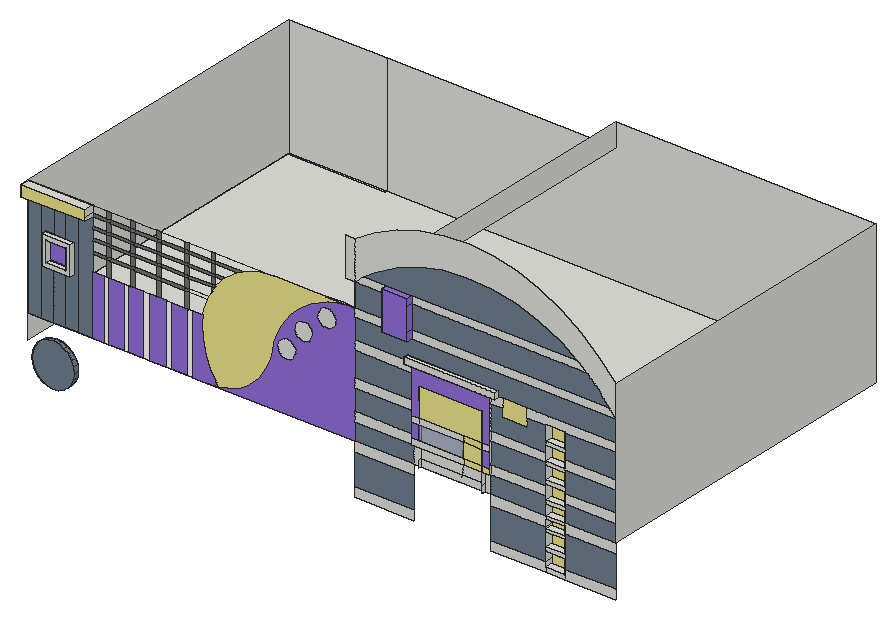
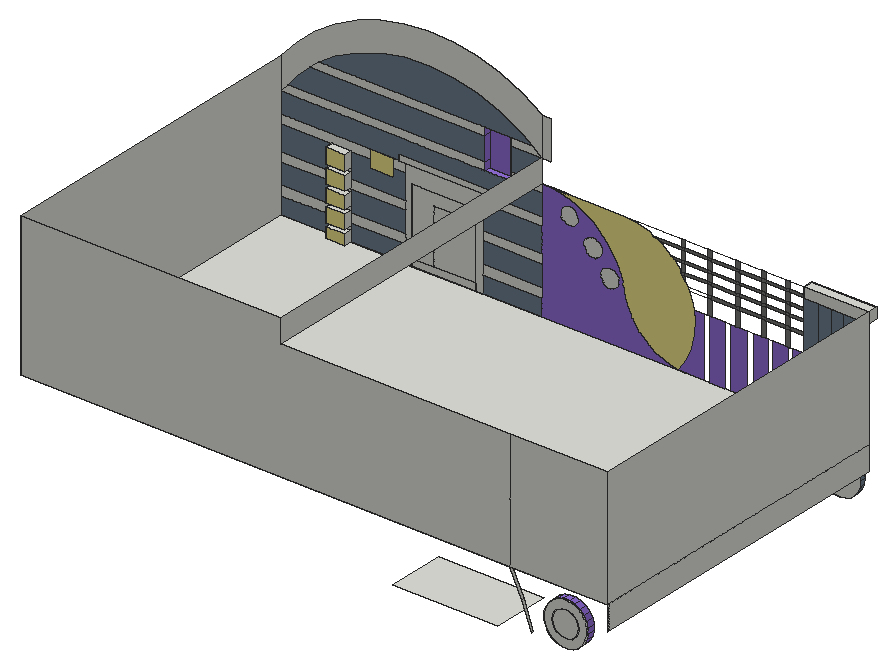
# SketchUp Ruby script. Lengths in inches.
U = 1.inch
M = Sketchup.active_model
def pt(a) = Geom::Point3d.new(a.map { |v| v * U })
def face(e, loops, mat)
  f = e.add_face(loops[0].map { |a| pt(a) })
  loops[1..].each { |l| e.add_face(l.map { |a| pt(a) }).erase! }
  f.material = f.back_material = mat if mat
  f
end
# faces: each face lists its corners as indices into pts; further lists are holes
def faces(e, pts, list, mat = nil) = list.each { |f| face(e, (f[0].is_a?(Array) ? f : [f]).map { |l| l.map { |i| pts[i] } }, mat) }
# xy, xz, yz: faces in a plane at the given z, y or x. An outline is a flat list of corners, or four numbers for a rectangle; further outlines are holes
def ring(l) = l.size == 4 ? [[l[0], l[1]], [l[2], l[1]], [l[2], l[3]], [l[0], l[3]]] : l.each_slice(2).to_a
def flat(e, list, mat, &to3) = list.each { |f| face(e, (f[0].is_a?(Array) ? f : [f]).map { |l| ring(l).map { |u, v| to3.(u, v) } }, mat) }
def xy(e, z, list, mat = nil) = flat(e, list, mat) { |x, y| [x, y, z] }
def xz(e, y, list, mat = nil) = flat(e, list, mat) { |x, z| [x, y, z] }
def yz(e, x, list, mat = nil) = flat(e, list, mat) { |y, z| [x, y, z] }
def lines(e, pts, list) = list.each { |a, b| e.add_line(pt(pts[a]), pt(pts[b])) }
# prism: a flat outline (further loops are holes) pulled along v
def prism(e, loops, v, mat = nil)
  f = face(e, loops, mat); d = Geom::Vector3d.new(v.map { |x| x * U })
  f.pushpull(f.normal.samedirection?(d) ? d.length : -d.length)
end
def box(e, o, s, mat = nil) = prism(e, [[o, [o[0] + s[0], o[1], o[2]], [o[0] + s[0], o[1] + s[1], o[2]], [o[0], o[1] + s[1], o[2]]]], [0, 0, s[2]], mat)
def at(x, y, z, deg = 0) = Geom::Transformation.translation(pt([x, y, z])) * Geom::Transformation.rotation(ORIGIN, Z_AXIS, deg.degrees)
def axes(o, x, y, z) = Geom::Transformation.new([*x, 0, *y, 0, *z, 0, *pt(o).to_a, 1])
def part(name) = M.definitions.add(name)
# library, detail: a bought-in or finely detailed component or shape, given as its bounding box
def library(name, o, s) = part(name).tap { |d| box(d.entities, o, s) }
def detail(e, o, s) = box(e.add_group.entities, o, s)
def put(e, d, t, mat = nil) = e.add_instance(d, t).tap { |i| i.material = mat if mat }
def group(e, t, mat = nil) = e.add_group.tap { |g| g.transformation = t; g.material = mat if mat }.entities
root = M.entities
M.materials.add("[0047_Khaki]").color = [240, 230, 140]
M.materials.add("[0111_SlateGray]").color = [112, 128, 144]
M.materials.add("[0115_MediumPurple]").color = [147, 112, 219]
M.materials.add("[Metal Seamed]").color = [118, 119, 115]
M.materials.add("[Translucent Glass Sky Reflection]").color = [126, 138, 183]
M.materials["[Translucent Glass Sky Reflection]"].alpha = 0.52
xy(root,99,[[81.125,144.5625,119.5625,165.625]])
xy(root,101.3125,[[231.02,45.625,238.14,48.4375]])
xy(root,103.03,[[231.02,45.625,238.14,48.4375]])
xy(root,108.37,[[231.02,45.625,238.14,48.4375]])
xy(root,109.71,[[231.02,45.625,238.14,48.4375]])
xy(root,114.67,[[231.02,45.625,238.14,48.4375]])
xy(root,115.6875,[[231.02,45.625,238.14,48.4375]])
xy(root,118.98,[[231.02,45.625,238.14,48.4375]])
xy(root,120,[[208.5625,44.5625,208.57,44.5625,208.57,45.625],[40.75,45.625,40.75,164.9375,76.51,164.9375,76.51,165.625,256.75,165.625,256.75,45.625,238.14,45.625,238.14,48.4375,231.02,48.4375,231.02,45.625,211.0625,45.625,211.0625,45.9375,182.75,45.9375,182.75,45.625],[182.75,45.625,185.24,45.9375],[185.24,45.625,208.57,45.9375],[208.57,45.625,211.0625,45.9375],
  [231.02,45.625,238.14,48.4375],[40.75,164.9375,76.51,165.625]])
xy(root,123.89,[[231.02,45.625,238.14,48.4375]])
xy(root,125.21,[[231.02,45.625,238.14,48.4375]])
xy(root,130.42,[[231.02,45.625,238.14,48.4375]])
xy(root,131.8125,[[231.02,45.625,238.14,48.4375]])
xy(root,136.6,[[231.02,45.625,238.14,48.4375]])
xy(root,137.97,[[231.02,45.625,238.14,48.4375]])
xy(root,138.5625,[[47.13,43.75,57.71,45.625]])
xy(root,140.1,[[48.67,43.75,56.17,45.625]])
xy(root,143.12,[[231.02,45.625,238.14,48.4375]])
xy(root,144.5,[[231.02,45.625,238.14,48.4375]])
xy(root,147.02,[[185.24,44.5625,186.69,45.625],[186.69,44.5625,208.57,45.625]])
xy(root,147.6,[[48.67,43.75,56.17,45.625]])
xy(root,149.13,[[47.13,43.75,57.71,45.625]])
xy(root,150.125,[[231.02,45.625,238.14,48.4375]])
xy(root,152.8125,[[180.25,44.125,182.75,45.625],[182.75,44.125,211.0625,44.5625],[211.0625,44.125,213.6875,45.625],[182.75,44.5625,211.0625,45.625]])
xy(root,155.0625,[[180.25,44.125,213.6875,45.625]])
xy(root,160.89,[[172.4,43.5,181.8125,45.625]],"[0115_MediumPurple]")
xy(root,163.75,[[40.75,42,64.49,45.625]])
xy(root,175.1,[[172.4,43.5,181.8125,45.625]],"[0115_MediumPurple]")
xz(root,42,[[40.75,159.875,64.49,160.08,64.49,163.75,40.75,163.75]],"[0047_Khaki]")
xz(root,43.5,[[172.4,160.89,181.8125,175.1]],"[0115_MediumPurple]")
xz(root,43.75,[[[47.13,138.5625,57.71,149.13],[48.67,140.1,56.17,147.6]]])
xz(root,44,[[51.27,99.26,53.3125,99.52,55.22,100.3,56.85,101.54,58.11,103.17,58.91,105.0625,59.18,107.1,58.92,109.14,58.14,111.04,56.9,112.68,55.28,113.9375,53.38,114.73,51.34,115.01,49.3,114.75,47.4,113.97,45.76,112.73,44.51,111.1,43.71,109.21,43.43,107.17,43.69,105.13,44.47,103.23,45.72,101.59,47.34,100.33,49.24,99.54]],"[0111_SlateGray]")
xz(root,44.125,[[180.25,152.8125,213.6875,155.0625]])
xz(root,44.5625,[[208.5625,120,208.57,120,208.57,122.49],[182.75,126.91,201.68,128.95],[182.75,134.36,185.24,136.41],[185.24,134.36,201.68,136.41],[208.57,134.36,211.0625,136.41]])
xz(root,44.5625,[[201.68,126.91,208.57,128.95],[208.57,126.91,211.0625,128.95],[201.68,128.95,208.57,134.36],[201.68,134.36,208.57,136.41],[185.24,136.41,208.57,147.02]],"[0047_Khaki]")
xz(root,44.5625,[[182.75,128.95,185.24,134.36],[208.57,128.95,211.0625,134.36],[182.75,136.41,185.24,136.41,185.24,147.02,208.57,147.02,208.57,136.41,211.0625,136.41,211.0625,152.8125,182.75,152.8125]],"[0115_MediumPurple]")
xz(root,44.5625,[[185.24,128.95,201.68,134.36]],"[Translucent Glass Sky Reflection]")
xz(root,45.625,[[51.27,99.26,49.24,99.54,47.34,100.33,45.72,101.59,44.47,103.23,43.69,105.13,43.43,107.17,43.71,109.21,44.51,111.1,45.76,112.73,47.4,113.97,49.3,114.75,51.34,115.01,53.38,114.73,55.28,113.9375,56.9,112.68,58.14,111.04,58.92,109.14,59.18,107.1,58.91,105.0625,58.11,103.17,56.85,101.54,55.22,100.3,53.3125,99.52],[160.75,101.3125,182.75,104.75],[211.0625,101.3125,231.02,104.75],[231.02,101.3125,238.14,103.03],[238.14,101.3125,256.75,104.75],
  [231.02,108.37,238.14,109.71],[231.02,114.67,238.14,115.6875],[160.75,116.3125,182.75,120],[211.0625,116.3125,231.02,120],[238.14,116.3125,256.75,120],
  [231.02,118.98,238.14,120],[182.75,120,182.75,152.8125,211.0625,152.8125,211.0625,120,208.57,120,208.57,147.02,185.24,147.02,185.24,120],[185.24,120,208.57,122.49],[185.24,122.49,200.8,142.51],[200.8,122.49,208.57,122.49,208.57,147.02,185.24,147.02,185.24,142.51,200.8,142.51],
  [231.02,123.89,238.14,125.21],[160.75,126.3125,182.75,129.75],[211.0625,126.3125,231.02,129.75],[238.14,126.3125,256.75,129.75],[231.02,130.42,238.14,131.8125],
  [231.02,136.6,238.14,137.97],[160.75,137.54,182.75,140.75],[211.0625,137.54,231.02,140.75],[238.14,137.54,256.75,140.75],[135.67,138.07,136.53,138.14,137.35,138.43,138.06,138.92,138.62,139.58,138.98,140.36,139.14,141.21,139.07,142.08,138.78,142.89,138.28,143.6,137.625,144.16,136.84,144.53,135.99,144.68,135.13,144.61,134.32,144.32,133.61,143.83,133.05,143.17,132.68,142.39,132.52,141.54,132.59,140.67,132.88,139.86,133.375,139.15,134.04,138.59,134.82,138.22],
  [[47.13,138.5625,57.71,149.13],[48.67,140.1,56.17,147.6]],[231.02,143.12,238.14,144.5],[141.94,146.02,142.8,146.09,143.62,146.38,144.33,146.87,144.89,147.53,145.26,148.3125,145.41,149.16,145.34,150.03,145.05,150.84,144.56,151.55,143.9,152.11,143.11,152.48,142.26,152.63,141.4,152.5625,140.59,152.27,139.875,151.78,139.32,151.12,138.95,150.34,138.79,149.49,138.86,148.625,139.16,147.81,139.65,147.1,140.31,146.54,141.09,146.17],[160.75,149.875,182.75,149.875,182.75,152.8125,180.25,152.8125,180.25,153.11,160.75,153.11],[211.0625,149.875,215.22,149.875,215.22,153.11,213.6875,153.11,213.6875,152.8125,211.0625,152.8125],
  [224.28,149.875,231.02,149.875,231.02,150.125,238.14,150.125,238.14,149.875,256.75,149.875,256.75,153.11,224.28,153.11],[180.25,152.8125,213.6875,155.0625],[150.53,153.47,151.39,153.54,152.21,153.83,152.92,154.33,153.48,154.99,153.85,155.77,154,156.62,153.93,157.48,153.64,158.29,153.15,159,152.49,159.5625,151.71,159.93,150.85,160.09,149.99,160.02,149.18,159.73,148.47,159.23,147.91,158.57,147.54,157.79,147.38,156.94,147.46,156.08,147.75,155.26,148.24,154.55,148.9,153.99,149.68,153.625],[40.75,159.875,40.75,163.75,64.49,163.75,64.49,160.08,50.125,159.96,45.3125,159.91],[160.75,160.89,172.4,163.75],
  [256.75,160.89,256.75,172.375,250.84,179.0625,244.13,184.94,236.72,189.93,228.74,193.93,220.32,196.88,211.59,198.74,202.7,199.48,193.78,199.08,184.99,197.55,176.46,194.92,168.34,191.22,160.75,186.53,160.75,172.375,164.37,175.1,167.99,177.82,175.92,182.21,184.38,185.46,193.21,187.51,202.24,188.32,211.29,187.87,220.19,186.17,228.77,183.26,236.87,179.18,242.78,175.1,244.32,174.03,246.12,172.375,250.99,167.89,254.4,163.75],[181.8125,160.89,256.75,160.89,254.4,163.75,181.8125,163.75],[150.22,163.75,160.75,163.75,156.39,164.07,152.03,163.97],[157.5625,172.375,160.75,186.53],[160.75,172.375,172.4,172.375,172.4,175.1,164.37,175.1],
  [181.8125,172.375,246.12,172.375,244.32,174.03,242.78,175.1,181.8125,175.1]])
xz(root,45.625,[[110.92,120.18,113.78,120.74,116.56,121.64,119.2,122.89,121.66,124.47,123.9,126.34,125.89,128.48,127.59,130.85,128.98,133.42,130.04,136.14,130.74,138.97,131.08,141.875,132.22,144.96,133.67,147.91,135.43,150.68,137.47,153.26,139.78,155.6,142.32,157.69,145.0625,159.5,147.98,161.01,151.05,162.2,154.22,163.06,157.47,163.58,160.75,163.75,131.08,163.75,126.1,163.28,121.29,161.87,119.97,161.19,117.79,160.08,116.84,159.59,113.35,156.86,112.89,156.5,112.43,155.98,109.94,153.12,109.6,152.73,109.23,152.11,108.25,150.41,107.08,148.41,106.78,147.58,105.41,143.6875,105.14,141.875,104.67,138.74,104.87,133.74,106.01,128.86,108.05,124.29],[215.22,146.8,224.28,153.11]],"[0047_Khaki]")
xz(root,45.625,[[160.75,104.75,182.75,116.3125],[211.0625,104.75,231.02,116.3125],[238.14,104.75,256.75,116.3125],[40.75,120,45.3125,120,45.3125,159.91,40.75,159.875],[45.3125,120,50.125,120,50.125,138.5625,47.13,138.5625,47.13,149.13,50.125,149.13,50.125,159.96,45.3125,159.91],
  [50.125,120,54.25,138.5625],[54.25,120,64.49,120,64.49,160.08,50.125,159.96,50.125,149.13,57.71,149.13,57.71,138.5625,54.25,138.5625],[160.75,120,182.75,126.3125],[211.0625,120,231.02,126.3125],[238.14,120,256.75,126.3125],
  [160.75,129.75,182.75,137.54],[211.0625,129.75,231.02,137.54],[238.14,129.75,256.75,137.54],[160.75,140.75,182.75,149.875],[211.0625,140.75,231.02,140.75,231.02,149.875,224.28,149.875,224.28,146.8,215.22,146.8,215.22,149.875,211.0625,149.875],
  [238.14,140.75,256.75,149.875],[160.75,153.11,180.25,153.11,180.25,155.0625,213.6875,155.0625,213.6875,153.11,256.75,153.11,256.75,160.89,160.75,160.89],[160.75,163.75,172.4,172.375],[181.8125,163.75,254.4,163.75,250.99,167.89,246.12,172.375,181.8125,172.375],[164.37,175.1,242.78,175.1,236.87,179.18,228.77,183.26,220.19,186.17,211.29,187.87,202.24,188.32,193.21,187.51,184.38,185.46,175.92,182.21,167.99,177.82]],"[0111_SlateGray]")
xz(root,45.625,[[64.49,120,68.69,141.875],[70.54,120,75.76,141.875],[77.65,120,82.98,141.875],[85.49,120,91.4,141.875],[93.75,120,99.21,141.875],
  [101.45,120,108,120,110.92,120.18,108.05,124.29,106.01,128.86,104.87,133.74,104.67,138.74,105.14,141.875,101.45,141.875],[[108,120,160.75,120,160.75,163.75,157.47,163.58,154.22,163.06,151.05,162.2,147.98,161.01,145.0625,159.5,142.32,157.69,139.78,155.6,137.47,153.26,135.43,150.68,133.67,147.91,132.22,144.96,131.08,141.875,130.74,138.97,130.04,136.14,128.98,133.42,127.59,130.85,125.89,128.48,123.9,126.34,121.66,124.47,119.2,122.89,116.56,121.64,113.78,120.74,110.92,120.18],[150.53,153.47,149.68,153.625,148.9,153.99,148.24,154.55,147.75,155.26,147.46,156.08,147.38,156.94,147.54,157.79,147.91,158.57,148.47,159.23,149.18,159.73,149.99,160.02,150.85,160.09,151.71,159.93,152.49,159.5625,153.15,159,153.64,158.29,153.93,157.48,154,156.62,153.85,155.77,153.48,154.99,152.92,154.33,152.21,153.83,151.39,153.54],[135.67,138.07,134.82,138.22,134.04,138.59,133.375,139.15,132.88,139.86,132.59,140.67,132.52,141.54,132.68,142.39,133.05,143.17,133.61,143.83,134.32,144.32,135.13,144.61,135.99,144.68,136.84,144.53,137.625,144.16,138.28,143.6,138.78,142.89,139.07,142.08,139.14,141.21,138.98,140.36,138.62,139.58,138.06,138.92,137.35,138.43,136.53,138.14],[141.94,146.02,141.09,146.17,140.31,146.54,139.65,147.1,139.16,147.81,138.86,148.625,138.79,149.49,138.95,150.34,139.32,151.12,139.875,151.78,140.59,152.27,141.4,152.5625,142.26,152.63,143.11,152.48,143.9,152.11,144.56,151.55,145.05,150.84,145.34,150.03,145.41,149.16,145.26,148.3125,144.89,147.53,144.33,146.87,143.62,146.38,142.8,146.09]],[48.67,140.1,56.17,147.6]],"[0115_MediumPurple]")
xz(root,45.625,[[69.84,141.875,71.23,147.58],[78.54,141.875,80,147.58],[88,141.875,89.49,147.58],[98.4,141.875,100.02,147.58],[64.49,147.58,69.84,148.74],
  [69.84,147.58,71.23,148.74],[71.23,147.58,78.54,148.74],[78.54,147.58,80,148.74],[80,147.58,88,148.74],[88,147.58,89.49,148.74],
  [89.49,147.58,98.4,148.74],[98.4,147.58,100.02,148.74],[69.84,148.74,71.23,152.11],[78.54,148.74,80,152.11],[88,148.74,89.49,152.11],
  [98.4,148.74,100.02,152.11],[108.25,150.41,109.23,152.11,108.25,152.11],[64.49,152.11,69.84,153.12],[69.84,152.11,71.23,153.12],[71.23,152.11,78.54,153.12],
  [78.54,152.11,80,153.12],[80,152.11,88,153.12],[88,152.11,89.49,153.12],[89.49,152.11,98.4,153.12],[98.4,152.11,100.02,153.12],
  [100.02,152.11,108.25,153.12],[108.25,152.11,109.23,153.12],[109.23,152.11,109.6,152.73,109.94,153.12,109.23,153.12],[69.84,153.12,71.23,155.98],[78.54,153.12,80,155.98],
  [88,153.12,89.49,155.98],[98.4,153.12,100.02,155.98],[108.25,153.12,109.23,155.98],[64.49,155.98,69.84,156.86],[69.84,155.98,71.23,156.86],
  [71.23,155.98,78.54,156.86],[78.54,155.98,80,156.86],[80,155.98,88,156.86],[88,155.98,89.49,156.86],[89.49,155.98,98.4,156.86],
  [98.4,155.98,100.02,156.86],[100.02,155.98,108.25,156.86],[108.25,155.98,109.23,156.86],[109.23,155.98,112.43,155.98,112.89,156.5,113.35,156.86,109.23,156.86],[69.84,156.86,71.23,160.08],
  [78.54,156.86,80,160.08],[88,156.86,89.49,160.08],[98.4,156.86,100.02,160.08],[108.25,156.86,109.23,160.08],[64.49,160.08,69.84,161.19],
  [69.84,160.08,71.23,161.19],[71.23,160.08,78.54,161.19],[78.54,160.08,80,161.19],[80,160.08,88,161.19],[88,160.08,89.49,161.19],
  [89.49,160.08,98.4,161.19],[98.4,160.08,100.02,161.19],[100.02,160.08,108.25,161.19],[108.25,160.08,109.23,161.19],[109.23,160.08,117.79,160.08,119.97,161.19,109.23,161.19],
  [69.84,161.19,71.23,163.75],[78.54,161.19,80,163.75],[88,161.19,89.49,163.75],[98.4,161.19,100.02,163.75],[108.25,161.19,109.23,163.75]],"[Metal Seamed]")
xz(root,48.4375,[[231.02,103.03,238.14,108.37],[231.02,109.71,238.14,114.67],[231.02,115.6875,238.14,118.98],[231.02,120,238.14,123.89],[231.02,125.21,238.14,130.42],
  [231.02,131.8125,238.14,136.6],[231.02,137.97,238.14,143.12],[231.02,144.5,238.14,150.125]],"[0047_Khaki]")
xz(root,162.1875,[[[55.29,100.3125,57.36,100.33,59.35,100.88,61.14,101.93,62.59,103.41,63.61,105.21,64.13,107.22,64.11,109.29,63.56,111.29,62.51,113.08,61.03,114.53,59.23,115.55,57.22,116.07,55.15,116.05,53.15,115.5,51.37,114.44,49.91,112.97,48.89,111.16,48.375,109.16,48.39,107.09,48.95,105.09,50,103.3,51.48,101.85,53.28,100.83],[56.25,103.3125,54.99,103.48,53.82,103.97,52.81,104.74,52.03,105.75,51.54,106.93,51.38,108.1875,51.54,109.45,52.03,110.625,52.81,111.64,53.82,112.41,54.99,112.9,56.25,113.0625,57.52,112.9,58.69,112.41,59.7,111.64,60.48,110.625,60.96,109.45,61.13,108.1875,60.96,106.93,60.48,105.75,59.7,104.74,58.69,103.97,57.52,103.48]]],"[0115_MediumPurple]")
xz(root,165.625,[[[55.29,100.3125,53.28,100.83,51.48,101.85,50,103.3,48.95,105.09,48.39,107.09,48.375,109.16,48.89,111.16,49.91,112.97,51.37,114.44,53.15,115.5,55.15,116.05,57.22,116.07,59.23,115.55,61.03,114.53,62.51,113.08,63.56,111.29,64.11,109.29,64.13,107.22,63.61,105.21,62.59,103.41,61.14,101.93,59.35,100.88,57.36,100.33],[56.25,103.3125,57.52,103.48,58.69,103.97,59.7,104.74,60.48,105.75,60.96,106.93,61.13,108.1875,60.96,109.45,60.48,110.625,59.7,111.64,58.69,112.41,57.52,112.9,56.25,113.0625,54.99,112.9,53.82,112.41,52.81,111.64,52.03,110.625,51.54,109.45,51.38,108.1875,51.54,106.93,52.03,105.75,52.81,104.74,53.82,103.97,54.99,103.48]],[56.25,103.3125,54.99,103.48,53.82,103.97,52.81,104.74,52.03,105.75,51.54,106.93,51.38,108.1875,51.54,109.45,52.03,110.625,52.81,111.64,53.82,112.41,54.99,112.9,56.25,113.0625,57.52,112.9,58.69,112.41,59.7,111.64,60.48,110.625,60.96,109.45,61.13,108.1875,60.96,106.93,60.48,105.75,59.7,104.74,58.69,103.97,57.52,103.48],[40.75,120,76.51,163.75],[76.51,120,76.51,163.75,160.75,163.75,160.75,172.375,256.75,172.375,256.75,120]])
yz(root,40.75,[[45.625,111.01,164.9375,120],[164.9375,111.01,165.625,120],[45.625,120,165.625,163.75],[42,159.875,45.625,163.75]])
yz(root,47.13,[[43.75,138.5625,45.625,149.13]])
yz(root,48.67,[[43.75,140.1,45.625,147.6]])
yz(root,56.17,[[43.75,140.1,45.625,147.6]])
yz(root,57.71,[[43.75,138.5625,45.625,149.13]])
yz(root,64.49,[[42,160.08,45.625,161.19],[42,161.19,45.625,163.75]])
yz(root,160.75,[[45.625,163.75,165.625,172.375]])
yz(root,172.4,[[43.5,160.89,45.625,163.75],[43.5,163.75,45.625,172.375],[43.5,172.375,45.625,175.1]],"[0115_MediumPurple]")
yz(root,180.25,[[44.125,152.8125,45.625,155.0625]])
yz(root,181.8125,[[43.5,160.89,45.625,163.75],[43.5,163.75,45.625,172.375],[43.5,172.375,45.625,175.1]],"[0115_MediumPurple]")
yz(root,185.24,[[44.5625,120,45.625,122.49],[44.5625,142.51,45.625,147.02]])
yz(root,208.57,[[44.5625,120,45.625,122.49],[44.5625,122.49,45.625,147.02]])
yz(root,213.6875,[[44.125,152.8125,45.625,155.0625]])
yz(root,231.02,[[45.625,103.03,48.4375,104.75],[45.625,104.75,48.4375,108.37],[45.625,109.71,48.4375,114.67],[45.625,115.6875,48.4375,116.3125],[45.625,116.3125,48.4375,118.98],
  [45.625,120,48.4375,123.89],[45.625,125.21,48.4375,130.42],[45.625,131.8125,48.4375,136.6],[45.625,137.97,48.4375,143.12],[45.625,144.5,48.4375,150.125]])
yz(root,238.14,[[45.625,103.03,48.4375,104.75],[45.625,104.75,48.4375,108.37],[45.625,109.71,48.4375,114.67],[45.625,115.6875,48.4375,116.3125],[45.625,116.3125,48.4375,118.98],
  [45.625,120,48.4375,123.89],[45.625,125.21,48.4375,130.42],[45.625,131.8125,48.4375,136.6],[45.625,137.97,48.4375,143.12],[45.625,144.5,48.4375,150.125]])
yz(root,256.75,[[45.625,120,165.625,172.375]])
p = [[49.24,45.625,99.54],[51.27,45.625,99.26],[51.27,44,99.26],[49.24,44,99.54],[53.3125,45.625,99.52],[53.3125,44,99.52],
  [47.34,45.625,100.33],[47.34,44,100.33],[55.22,45.625,100.3],[55.22,44,100.3],[45.72,45.625,101.59],[45.72,44,101.59],
  [56.85,45.625,101.54],[56.85,44,101.54],[53.28,162.1875,100.83],[53.28,164.9375,100.83],[55.29,164.9375,100.3125],[55.29,162.1875,100.3125],
  [57.36,164.9375,100.33],[57.36,162.1875,100.33],[59.35,164.9375,100.88],[59.35,162.1875,100.88],[53.28,165.625,100.83],[55.29,165.625,100.3125],
  [57.36,165.625,100.33],[59.35,165.625,100.88],[51.48,162.1875,101.85],[51.48,164.9375,101.85],[51.48,165.625,101.85],[68.66,165.625,100.82],
  [72.21,165.625,110.5625],[72.21,164.9375,110.5625],[68.66,164.9375,100.82],[61.14,164.9375,101.93],[61.14,162.1875,101.93],[61.14,165.625,101.93],
  [58.11,45.625,103.17],[58.11,44,103.17],[44.47,45.625,103.23],[44.47,44,103.23],[50,162.1875,103.3],[50,164.9375,103.3],
  [62.59,164.9375,103.41],[62.59,162.1875,103.41],[50,165.625,103.3],[62.59,165.625,103.41],[43.69,45.625,105.13],[43.69,44,105.13],
  [58.91,45.625,105.0625],[58.91,44,105.0625],[48.95,162.1875,105.09],[48.95,164.9375,105.09],[56.25,165.625,103.3125],[54.99,165.625,103.48],
  [54.99,162.1875,103.48],[56.25,162.1875,103.3125],[57.52,165.625,103.48],[57.52,162.1875,103.48],[48.95,165.625,105.09],[63.61,164.9375,105.21],
  [63.61,162.1875,105.21],[63.61,165.625,105.21],[53.82,165.625,103.97],[53.82,162.1875,103.97],[58.69,165.625,103.97],[58.69,162.1875,103.97],
  [52.81,165.625,104.74],[52.81,162.1875,104.74],[59.7,165.625,104.74],[59.7,162.1875,104.74],[52.03,165.625,105.75],[52.03,162.1875,105.75],
  [60.48,165.625,105.75],[60.48,162.1875,105.75],[43.43,45.625,107.17],[43.43,44,107.17],[59.18,45.625,107.1],[59.18,44,107.1],
  [48.39,162.1875,107.09],[48.39,164.9375,107.09],[48.39,165.625,107.09],[64.13,164.9375,107.22],[64.13,162.1875,107.22],[64.13,165.625,107.22],
  [51.54,165.625,106.93],[51.54,162.1875,106.93],[60.96,165.625,106.93],[60.96,162.1875,106.93],[51.38,165.625,108.1875],[51.38,162.1875,108.1875],
  [61.13,165.625,108.1875],[61.13,162.1875,108.1875],[58.92,45.625,109.14],[58.92,44,109.14],[48.375,162.1875,109.16],[48.375,164.9375,109.16],
  [48.375,165.625,109.16],[43.71,45.625,109.21],[43.71,44,109.21],[64.11,164.9375,109.29],[64.11,162.1875,109.29],[64.11,165.625,109.29],
  [51.54,165.625,109.45],[51.54,162.1875,109.45],[60.96,165.625,109.45],[60.96,162.1875,109.45],[58.14,45.625,111.04],[58.14,44,111.04],
  [44.51,45.625,111.1],[44.51,44,111.1],[48.89,162.1875,111.16],[48.89,164.9375,111.16],[48.89,165.625,111.16],[63.56,164.9375,111.29],
  [63.56,162.1875,111.29],[63.56,165.625,111.29],[52.03,165.625,110.625],[52.03,162.1875,110.625],[60.48,165.625,110.625],[60.48,162.1875,110.625],
  [52.81,165.625,111.64],[52.81,162.1875,111.64],[59.7,165.625,111.64],[59.7,162.1875,111.64],[76.51,165.625,120],[76.51,164.9375,120],
  [56.9,45.625,112.68],[56.9,44,112.68],[45.76,45.625,112.73],[45.76,44,112.73],[49.91,162.1875,112.97],[49.91,164.9375,112.97],
  [49.91,165.625,112.97],[62.51,164.9375,113.08],[62.51,162.1875,113.08],[62.51,165.625,113.08],[53.82,165.625,112.41],[53.82,162.1875,112.41],
  [58.69,165.625,112.41],[58.69,162.1875,112.41],[54.99,165.625,112.9],[54.99,162.1875,112.9],[57.52,165.625,112.9],[57.52,162.1875,112.9],
  [47.4,45.625,113.97],[47.4,44,113.97],[55.28,45.625,113.9375],[55.28,44,113.9375],[56.25,165.625,113.0625],[56.25,162.1875,113.0625],
  [51.37,162.1875,114.44],[51.37,164.9375,114.44],[51.37,165.625,114.44],[61.03,164.9375,114.53],[61.03,162.1875,114.53],[61.03,165.625,114.53],
  [53.38,45.625,114.73],[53.38,44,114.73],[49.3,45.625,114.75],[49.3,44,114.75],[53.15,162.1875,115.5],[53.15,164.9375,115.5],
  [53.15,165.625,115.5],[59.23,164.9375,115.55],[59.23,162.1875,115.55],[59.23,165.625,115.55],[51.34,45.625,115.01],[51.34,44,115.01],
  [55.15,162.1875,116.05],[55.15,164.9375,116.05],[57.22,164.9375,116.07],[57.22,162.1875,116.07],[55.15,165.625,116.05],[57.22,165.625,116.07],
  [40.75,45.625,159.875],[45.3125,45.625,159.91],[50.125,45.625,159.96],[64.49,45.625,160.08],[64.49,42,160.08],[40.75,42,159.875],
  [131.08,45.625,163.75],[109.23,45.625,163.75],[69.84,45.625,163.75],[64.49,45.625,163.75],[78.54,45.625,163.75],[71.23,45.625,163.75],
  [88,45.625,163.75],[80,45.625,163.75],[98.4,45.625,163.75],[89.49,45.625,163.75],[100.02,45.625,147.58],[106.78,45.625,147.58],
  [100.02,45.625,148.74],[107.08,45.625,148.74],[108.25,45.625,163.75],[100.02,45.625,163.75],[54.25,45.625,149.13],[54.25,45.625,159.96],
  [59.17,45.625,120],[59.17,45.625,159.96],[100.02,45.625,141.875],[101.45,45.625,141.875],[68.69,45.625,141.875],[69.84,45.625,141.875],
  [75.76,45.625,141.875],[77.65,45.625,141.875],[82.98,45.625,141.875],[85.49,45.625,141.875],[91.4,45.625,141.875],[93.75,45.625,141.875],
  [200.8,45.625,122.49],[200.8,44.5625,122.49]]
faces(root,p,[[0,1,2,3],[1,4,5,2],[6,0,3,7],[4,8,9,5],[10,6,7,11],[8,12,13,9],[12,36,37,13],[38,10,11,39],
  [46,38,39,47],[36,48,49,37],[74,46,47,75],[48,76,77,49],[76,92,93,77],[97,74,75,98],[92,106,107,93],[108,97,98,109],
  [106,126,127,107],[128,108,109,129],[144,128,129,145],[126,146,147,127],[146,156,157,147],[158,144,145,159],[156,166,167,157],[166,158,159,167]],"[0111_SlateGray]")
faces(root,p,[[14,15,16,17],[17,16,18,19],[19,18,20,21],[26,27,15,14],[21,20,33,34],[40,41,27,26],[34,33,42,43],[50,51,41,40],
  [43,42,59,60],[78,79,51,50],[60,59,81,82],[94,95,79,78],[82,81,99,100],[110,111,95,94],[100,99,113,114],[130,131,111,110],
  [114,113,133,134],[150,151,131,130],[134,133,153,154],[160,161,151,150],[154,153,163,164],[168,169,161,160],[164,163,170,171],[171,170,169,168]],"[0115_MediumPurple]")
faces(root,p,[[22,23,16,15],[23,24,18,16],[24,25,20,18],[28,22,15,27],[29,30,31,32],[25,35,33,20],[44,28,27,41],[35,45,42,33],
  [52,53,54,55],[56,52,55,57],[58,44,41,51],[45,61,59,42],[53,62,63,54],[64,56,57,65],[62,66,67,63],[68,64,65,69],
  [66,70,71,67],[72,68,69,73],[80,58,51,79],[61,83,81,59],[70,84,85,71],[86,72,73,87],[84,88,89,85],[90,86,87,91],
  [96,80,79,95],[83,101,99,81],[88,102,103,89],[104,90,91,105],[112,96,95,111],[101,115,113,99],[102,116,117,103],[118,104,105,119],
  [116,120,121,117],[122,118,119,123],[30,124,125,31],[132,112,111,131],[115,135,133,113],[120,136,137,121],[138,122,123,139],[136,140,141,137],
  [142,138,139,143],[140,148,149,141],[148,142,143,149],[152,132,131,151],[135,155,153,133],[162,152,151,161],[155,165,163,153],[172,162,161,169],
  [165,173,170,163],[173,172,169,170],[174,175,176,177,178,179]])
lines(root,p,[[180,181],[182,183],[184,185],[186,187],[188,189],[190,191],[192,193],[194,195],[196,197],[198,199],[200,201],[202,203],
  [204,205],[206,207],[208,209],[210,211]])
